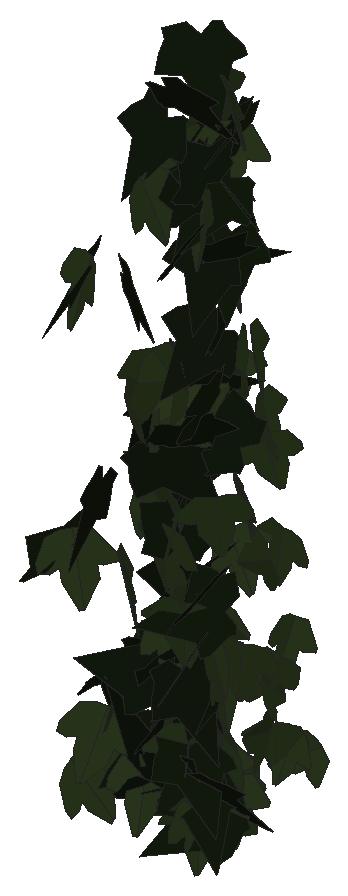
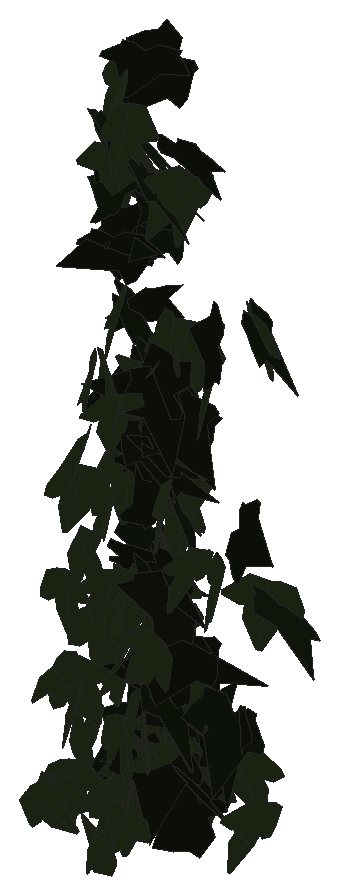
# SketchUp Ruby script. Lengths in inches.
U = 1.inch
M = Sketchup.active_model
def pt(a) = Geom::Point3d.new(a.map { |v| v * U })
def face(e, loops, mat)
  f = e.add_face(loops[0].map { |a| pt(a) })
  loops[1..].each { |l| e.add_face(l.map { |a| pt(a) }).erase! }
  f.material = f.back_material = mat if mat
  f
end
# faces: each face lists its corners as indices into pts; further lists are holes
def faces(e, pts, list, mat = nil) = list.each { |f| face(e, (f[0].is_a?(Array) ? f : [f]).map { |l| l.map { |i| pts[i] } }, mat) }
# xy, xz, yz: faces in a plane at the given z, y or x. An outline is a flat list of corners, or four numbers for a rectangle; further outlines are holes
def ring(l) = l.size == 4 ? [[l[0], l[1]], [l[2], l[1]], [l[2], l[3]], [l[0], l[3]]] : l.each_slice(2).to_a
def flat(e, list, mat, &to3) = list.each { |f| face(e, (f[0].is_a?(Array) ? f : [f]).map { |l| ring(l).map { |u, v| to3.(u, v) } }, mat) }
def xy(e, z, list, mat = nil) = flat(e, list, mat) { |x, y| [x, y, z] }
def xz(e, y, list, mat = nil) = flat(e, list, mat) { |x, z| [x, y, z] }
def yz(e, x, list, mat = nil) = flat(e, list, mat) { |y, z| [x, y, z] }
def lines(e, pts, list) = list.each { |a, b| e.add_line(pt(pts[a]), pt(pts[b])) }
# prism: a flat outline (further loops are holes) pulled along v
def prism(e, loops, v, mat = nil)
  f = face(e, loops, mat); d = Geom::Vector3d.new(v.map { |x| x * U })
  f.pushpull(f.normal.samedirection?(d) ? d.length : -d.length)
end
def box(e, o, s, mat = nil) = prism(e, [[o, [o[0] + s[0], o[1], o[2]], [o[0] + s[0], o[1] + s[1], o[2]], [o[0], o[1] + s[1], o[2]]]], [0, 0, s[2]], mat)
def at(x, y, z, deg = 0) = Geom::Transformation.translation(pt([x, y, z])) * Geom::Transformation.rotation(ORIGIN, Z_AXIS, deg.degrees)
def axes(o, x, y, z) = Geom::Transformation.new([*x, 0, *y, 0, *z, 0, *pt(o).to_a, 1])
def part(name) = M.definitions.add(name)
# library, detail: a bought-in or finely detailed component or shape, given as its bounding box
def library(name, o, s) = part(name).tap { |d| box(d.entities, o, s) }
def detail(e, o, s) = box(e.add_group.entities, o, s)
def put(e, d, t, mat = nil) = e.add_instance(d, t).tap { |i| i.material = mat if mat }
def group(e, t, mat = nil) = e.add_group.tap { |g| g.transformation = t; g.material = mat if mat }.entities
root = M.entities
M.materials.add("efeu1").color = [18, 25, 13]
M.materials.add("efeu2").color = [43, 57, 29]
c1 = part("ivyleaf_9")
p = [[1.54,2.16,1.25],[1.36,2.04,1.19],[-0.21,0.99,0.68],[-0.71,1.11,0.82],[-0.85,0.86,0.67],[-0.8,0.17,0.21],
  [-0.9,-0.01,0.1],[-0.67,-0.16,-0.02],[-0.08,-0.08,-0.05],[-0.03,-0.6,-0.4],[0.65,-0.88,-0.66],[0.83,-0.6,-0.49],
  [1.29,-0.42,-0.43],[1.8125,-0.07,-0.26],[1.21,0.44,0.15]]
faces(c1.entities,p,[[0,1,2,3,4,5,6,7,8,9,10,11,12,13,14]],"efeu1")
c2 = part("ivyleaf_10")
p = [[0,0.5,-0.03],[-0.0625,2.02,-0.43],[-0.19,2.01,-0.46],[-0.54,1.05,-0.29],[-0.52,0.625,-0.18],[-0.83,0.76,-0.28],
  [-1.16,0.64,-0.33],[-1.15,0.33,-0.24],[-0.77,-0.39,0.02],[-0.3,-0.51,0.16],[0.04,-0.48,0.23],[-0.02,2.01,-0.4375],
  [-0.06,2.01,-0.43],[0.04,-0.49,0.23],[0.67,-0.49,0.14],[1.38,0.36,-0.2],[1.375,0.51,-0.24],[0.81,0.65,-0.19],
  [0.62,0.59,-0.15],[0.6,1.09,-0.28],[0.5,1.23,-0.31]]
faces(c2.entities,p,[[0,1,2,3,4,5,6,7,8,9,10],[11,12,0,13,14,15,16,17,18,19,20]],"efeu2")
put(root,c1,axes([599.48,135.08,196.09],[-0.17515,0.56186,0.50454],[-0.19533,0.4666,-0.58741],[-0.72945,-0.25986,0.03615]))
put(root,c2,axes([598.03,135.5,191.97],[-0.83142,0.16967,0.09937],[-0.11258,-0.05682,-0.845],[-0.1612,-0.83541,0.07765]))
put(root,c2,axes([597.29,135.13,195.71],[-0.33542,0.39582,0.64097],[-0.41193,0.49108,-0.51882],[-0.63074,-0.53122,-0.00202]))
put(root,c1,axes([598.03,135.34,194.51],[-0.09921,-0.26302,-0.75239],[0.1878,0.72913,-0.27966],[0.77459,-0.21047,-0.02857]))
put(root,c1,axes([598.74,135.27,195.4],[0.4239,0.64776,-0.12364],[-0.07765,-0.09693,-0.77404],[-0.65486,0.43079,0.01175]))
put(root,c1,axes([598.58,135.89,185.9375],[0.02815,-0.77163,-0.17513],[0.1769,0.17695,-0.75118],[0.77123,-0.01242,0.1787]))
put(root,c2,axes([597.77,135.55,196.91],[-0.60445,-0.48908,-0.20865],[0.17064,0.12078,-0.77743],[0.50361,-0.62794,0.01298]))
put(root,c1,axes([598.28,135.375,204.74],[0.79843,0.15118,0.0487],[0.04798,0.00835,-0.81262],[-0.15141,0.79987,-0.00073]))
put(root,c1,axes([597.47,135.74,187.67],[-0.46495,0.1516,0.60854],[-0.58334,0.17358,-0.48894],[-0.23025,-0.7459,0.0099]))
put(root,c1,axes([599.15,135.2,190.59],[-0.05658,0.74396,0.27596],[-0.0347,0.27407,-0.746],[-0.79273,-0.06509,0.01296]))
put(root,c2,axes([597.77,135.15,196.43],[-0.10669,-0.23752,-0.78971],[0.33307,0.71605,-0.26036],[0.75441,-0.34972,0.00326]))
put(root,c1,axes([595.51,136.1,192.29],[-0.21723,0.20492,-0.73112],[0.53933,-0.49364,-0.2986],[-0.53447,-0.58142,-0.00416]))
put(root,c2,axes([597.76,136.12,190.25],[0.214,-0.2507,-0.71753],[0.44642,-0.56185,0.32945],[-0.61515,-0.49495,-0.01054]))
put(root,c1,axes([598.64,135.09,188.23],[0.12071,0.46617,0.65874],[0.01962,0.66418,-0.47361],[-0.80676,0.0859,0.08704]))
put(root,c2,axes([595.14,135.88,198.32],[0.69254,-0.41807,0.0234],[0.02287,-0.00739,-0.80893],[0.4181,0.6929,0.0055]))
put(root,c1,axes([598.91,136.32,197.7],[-0.39809,-0.60806,0.27911],[-0.14546,-0.23836,-0.72674],[0.65306,-0.42375,0.00827]))
put(root,c2,axes([598.62,135.35,196.51],[0.0499,-0.09413,-0.86374],[-0.53865,0.67548,-0.10473],[0.68173,0.54061,-0.01953]))
put(root,c1,axes([595.23,135.91,198.4],[-0.585,0.44066,-0.32599],[0.25378,-0.20485,-0.73233],[-0.48584,-0.6376,0.00999]))
put(root,c2,axes([598.9,135.93,184.54],[-0.25955,-0.79481,0.09066],[-0.00821,-0.09266,-0.83586],[0.79992,-0.25884,0.02083]))
put(root,c1,axes([599.375,136,190.09],[-0.69551,0.10376,0.4092],[-0.41383,-0.01181,-0.70039],[-0.08338,-0.80687,0.06287]))
put(root,c1,axes([598.72,136.06,184.94],[-0.06841,-0.75084,-0.2086],[0.16447,0.19078,-0.74061],[0.76172,-0.10862,0.14118]))
put(root,c2,axes([598.46,135.8,189.77],[-0.77585,-0.31539,0.09171],[-0.075,-0.05893,-0.83709],[0.31977,-0.77902,0.02619]))
put(root,c2,axes([598.9375,135.75,184.42],[0.31576,0.78872,-0.0383],[-0.1311,0.01168,-0.84019],[-0.77869,0.31786,0.12592]))
put(root,c2,axes([598.68,136.05,201.31],[0.63049,-0.31526,0.33383],[0.2973,-0.15187,-0.70491],[0.34992,0.69706,-0.00259]))
put(root,c2,axes([597.98,135.73,192.43],[0.49156,-0.52468,-0.39049],[-0.26546,0.28639,-0.71897],[0.59775,0.55866,0.00183]))
put(root,c2,axes([598.41,135.92,186.31],[-0.44957,-0.657,0.04508],[0.04346,-0.08407,-0.79173],[0.65711,-0.44393,0.08321]))
put(root,c2,axes([594.93,135.72,190.5],[0.7318,0.39439,0.16682],[0.07748,0.20292,-0.81959],[-0.42115,0.72263,0.1391]))
put(root,c1,axes([599.31,136.27,184.27],[-0.69308,-0.25006,0.34141],[-0.3081,-0.15097,-0.73603],[0.29011,-0.75772,0.03397]))
put(root,c2,axes([596.51,135.82,190.39],[-0.53032,0.65007,-0.14118],[0.06273,-0.13088,-0.83827],[-0.66226,-0.53296,0.03365]))
put(root,c1,axes([598.33,135.89,187.99],[0.16995,-0.72031,-0.40589],[-0.09788,0.39394,-0.74007],[0.82098,0.19607,-0.00421]))
put(root,c2,axes([598.01,135.7,192.46],[-0.30314,0.13366,-0.74242],[-0.67019,0.31957,0.33117],[0.34628,0.7355,-0.00897]))
put(root,c1,axes([597.74,135.98,184.44],[0.55605,-0.4331,0.90783],[-0.70662,0.57003,0.70476],[-0.71583,-0.89912,0.00951]))
put(root,c2,axes([597.35,135.65,201.41],[0.02179,0.75819,0.25552],[-0.04629,0.25638,-0.7568],[-0.79875,0.00582,0.05083]))
put(root,c2,axes([598.02,136.11,185.84],[0.6614,-0.50269,0.10098],[0.08148,-0.05968,-0.83075],[0.50622,0.6664,0.00177]))
put(root,c2,axes([597.89,135.92,195.04],[0.12927,0.79092,-0.04758],[-0.01141,-0.04634,-0.8014],[-0.79227,0.12971,0.00378]))
put(root,c2,axes([596.87,136.05,184.62],[0.79945,0.05348,0.06015],[0.06007,0.00311,-0.80124],[-0.05357,0.80171,-0.0009]))
put(root,c2,axes([598.08,135.74,195.3125],[0.44704,0.04825,-0.66928],[0.64371,0.19622,0.44411],[0.18945,-0.78056,0.07027]))
put(root,c1,axes([598.49,135.35,200.05],[0.17816,0.49731,0.59196],[0.07371,0.59378,-0.52102],[-0.76961,0.17199,0.08713]))
put(root,c2,axes([595.47,136.13,185.53],[0.77809,0.23006,-0.17094],[-0.16674,-0.03892,-0.81133],[-0.23312,0.7957,0.00974]))
put(root,c1,axes([598.34,135.72,191.85],[-0.41721,-0.32068,0.67833],[0.53805,0.41307,0.52621],[-0.52294,0.68085,0.00024]))
put(root,c2,axes([599.2,136.0625,192.94],[-0.57017,-0.53486,-0.04718],[0.03496,0.0317,-0.78178],[0.5358,-0.57124,0.0008]))
put(root,c1,axes([597.87,135.91,186.68],[-0.27729,0.78448,-0.14614],[0.06048,-0.1336,-0.83195],[-0.79568,-0.28354,-0.01231]))
put(root,c1,axes([598.78,136.51,199.88],[-0.2675,-0.71367,0.01173],[-0.0042,-0.01096,-0.76215],[0.71375,-0.26753,-0.00009]))
put(root,c2,axes([597.36,136.02,187.1],[-0.74119,0.1043,-0.17165],[0.17063,-0.01923,-0.74848],[-0.10596,-0.76056,-0.00461]))
put(root,c1,axes([599.14,135.71,202.32],[-0.13653,0.53416,0.54564],[-0.41867,0.41118,-0.50728],[-0.63856,-0.38379,0.21593]))
put(root,c1,axes([594.48,135.73,190.2],[-0.24482,0.73594,0.3292],[-0.32043,0.22688,-0.7455],[-0.7398,-0.34181,0.21396]))
put(root,c1,axes([598.68,135.99,201.83],[-0.51041,0.43494,0.41114],[-0.35354,0.21689,-0.66835],[-0.48292,-0.61848,0.05475]))
put(root,c1,axes([597.25,136.46,203.02],[-0.71954,-0.19735,-0.20147],[0.20001,0.03213,-0.74581],[0.19882,-0.74652,0.02116]))
put(root,c1,axes([598.75,135.8,185.07],[0.82989,0.15234,0.10307],[0.08699,0.09458,-0.84026],[-0.16206,0.8309,0.07675]))
put(root,c2,axes([599.08,136.03,189.03],[-0.2248,0.70811,0.06754],[-0.01675,0.06554,-0.74293],[-0.71113,-0.22539,-0.00385]))
put(root,c1,axes([597.89,135.75,192.38],[-0.28954,0.59237,0.494],[-0.19526,0.45418,-0.65907],[-0.7462,-0.3487,-0.01922]))
put(root,c2,axes([597.64,136.22,189.02],[0.36369,0.69944,-0.01687],[-0.00786,-0.01492,-0.78834],[-0.6996,0.36377,0.00009]))
put(root,c2,axes([595.05,135.89,184.05],[0.09385,0.7266,0.41294],[0.04741,0.41024,-0.73262],[-0.8344,0.10504,0.00482]))
put(root,c1,axes([598.66,136.4,187.22],[-0.72112,0.37351,-0.01669],[-0.04987,-0.13203,-0.79993],[-0.37054,-0.70913,0.14014]))
put(root,c2,axes([597.77,136.02,190.68],[-0.57427,0.4899,0.28609],[-0.22552,0.17641,-0.75476],[-0.52056,-0.61686,0.01137]))
put(root,c2,axes([597.76,136.26,186.46],[-0.10204,0.73817,-0.0861],[0.00139,-0.08672,-0.74512],[-0.74318,-0.10152,0.01042]))
put(root,c1,axes([599,136.72,201.83],[-0.67768,-0.409,-0.01842],[0.01637,0.00852,-0.79154],[0.40909,-0.67788,0.00117]))
put(root,c1,axes([597.48,136.37,195.17],[-0.03756,0.59258,-0.4817],[-0.12238,-0.48072,-0.58183],[-0.7538,0.04852,0.11847]))
put(root,c1,axes([598.99,136.58,197.98],[-0.59621,0.31029,-0.35451],[0.27458,-0.23579,-0.66816],[-0.38284,-0.65234,0.07288]))
put(root,c1,axes([598.08,136.25,190.4],[-0.16878,0.01522,-0.77787],[-0.76448,-0.15106,0.16292],[-0.14448,0.7815,0.04664]))
put(root,c1,axes([598.17,136.32,193.31],[-0.43099,0.24942,0.60677],[-0.52164,0.30999,-0.49794],[-0.39785,-0.67664,-0.00445]))
put(root,c1,axes([595.75,136.15,186.64],[0.45284,0.09373,-0.6358],[-0.64167,0.02251,-0.4537],[-0.03588,0.78026,0.08946]))
put(root,c1,axes([599.38,136.63,194.51],[-0.23304,0.09191,0.72797],[-0.73365,-0.01646,-0.23278],[-0.01222,-0.76418,0.09257]))
put(root,c1,axes([597.4,136.03,187.26],[0.26049,0.06632,0.71485],[0.65229,0.29578,-0.26514],[-0.29988,0.70099,0.04424]))
put(root,c1,axes([598.5,136.6,185.51],[-0.72874,0.30952,0.03809],[-0.0838,-0.1011,-0.78171],[-0.30039,-0.72269,0.12567]))
put(root,c1,axes([597.17,136.04,188.47],[0.66728,0.50259,0.04955],[0.04373,0.02431,-0.83535],[-0.50313,0.66867,-0.00688]))
put(root,c1,axes([595.76,136.78,197.875],[0.20868,-0.06172,-0.74778],[0.74688,-0.05708,0.21315],[-0.07169,-0.77425,0.04389]))
put(root,c1,axes([596.57,136.3,183.66],[0.48787,0.58664,-0.32179],[0.21106,0.24299,0.76297],[0.63494,-0.53153,-0.00636]))
put(root,c1,axes([598.18,136.71,205.57],[-0.28676,-0.5517,-0.47132],[0.3021,0.37,-0.61691],[0.65973,-0.40923,0.07762]))
put(root,c2,axes([599.05,136.66,184.18],[0.47922,-0.00739,-0.60101],[-0.60031,0.03252,-0.47905],[0.03003,0.76799,0.0145]))
put(root,c2,axes([598.49,136.8,189.56],[-0.11099,0.04369,-0.73699],[0.65061,-0.34649,-0.11853],[-0.34897,-0.65987,0.01344]))
put(root,c1,axes([597.85,136.42,195.88],[-0.00056,0.76781,-0.18396],[0.00633,-0.18395,-0.76779],[-0.78952,-0.00202,-0.00602]))
put(root,c2,axes([595.67,136.48,185.62],[0.25176,-0.65765,0.35181],[-0.1295,0.32712,0.70418],[-0.73451,-0.28309,-0.00357]))
put(root,c2,axes([598.28,137.11,184],[-0.2401,0.20508,0.71295],[0.53247,-0.47415,0.31571],[0.51657,0.58406,0.00595]))
put(root,c2,axes([598.26,136.77,184.53],[-0.5946,-0.16977,0.33654],[-0.30668,-0.14756,-0.61628],[0.21915,-0.66711,0.05067]))
put(root,c1,axes([597.75,136.5,187.15],[-0.37506,0.71976,-0.00582],[-0.00081,-0.00699,-0.81161],[-0.71979,-0.37504,0.00395]))
put(root,c1,axes([597.43,136.19,189.52],[-0.06163,0.78621,-0.26039],[-0.02428,0.25928,0.78861],[0.82785,0.06614,0.00375]))
put(root,c1,axes([597.59,136.42,195.69],[0.3779,0.04918,0.66035],[0.65023,0.11624,-0.38076],[-0.12524,0.7519,0.01567]))
put(root,c2,axes([597.29,136.74,185.47],[0.42994,0.68079,-0.01207],[-0.04069,0.01144,-0.80417],[-0.67968,0.42996,0.0405]))
put(root,c1,axes([598.25,136.81,194.77],[-0.36857,0.59985,-0.325],[0.17966,-0.27102,-0.70396],[-0.65816,-0.4099,-0.01017]))
put(root,c2,axes([599,136.73,204.46],[-0.57255,0.54729,-0.1407],[0.1116,-0.08684,-0.79192],[-0.55395,-0.58315,-0.01411]))
put(root,c1,axes([598.8,136.25,199.6875],[0.44997,0.29569,0.54471],[0.40899,0.36412,-0.5355],[-0.4657,0.60548,0.05602]))
put(root,c1,axes([596.6875,136.92,184.98],[-0.76098,0.23429,0.0636],[-0.06777,-0.00408,-0.79587],[-0.23312,-0.76362,0.02377]))
put(root,c1,axes([598.83,137.07,200.05],[-0.41992,-0.53417,-0.34372],[0.28547,0.20938,-0.67415],[0.56744,-0.50064,0.08479]))
put(root,c2,axes([599.45,136.8,188.59],[-0.72286,-0.31484,0.13087],[-0.12968,-0.02985,-0.78808],[0.31533,-0.734,-0.02408]))
put(root,c2,axes([598.83,136.83,185.57],[-0.71162,0.2824,0.22154],[-0.2777,-0.12153,-0.73712],[-0.2274,-0.73534,0.2069]))
put(root,c2,axes([598.74,136.83,183.77],[-0.69527,-0.32853,0.09744],[-0.09468,-0.02766,-0.76883],[0.32934,-0.70152,-0.01532]))
put(root,c1,axes([599.03,136.87,203.24],[-0.5316,0.55983,-0.11159],[0.02452,-0.12995,-0.76875],[-0.57032,-0.52742,0.07097]))
put(root,c1,axes([595.61,136.37,186.96],[0.17098,0.77501,0.18738],[-0.06267,0.20411,-0.78701],[-0.79487,0.15061,0.10236]))
put(root,c2,axes([599,136.47,188.35],[0.23411,-0.2473,0.67716],[-0.41935,0.53241,0.33941],[-0.58639,-0.47948,0.02762]))
put(root,c2,axes([598.68,136.95,187.62],[-0.09386,0.71736,-0.13127],[0.02188,-0.12953,-0.72346],[-0.72894,-0.09626,-0.00481]))
put(root,c1,axes([598.42,137.125,193.93],[-0.54657,0.07563,0.53038],[-0.5292,0.04185,-0.55132],[-0.08348,-0.76045,0.0224]))
put(root,c1,axes([598.375,137.32,201.66],[0.28736,-0.59697,0.37739],[0.31687,-0.25515,-0.64488],[0.63119,0.39987,0.15193]))
put(root,c1,axes([597.51,136.78,185.42],[0.47694,0.59197,-0.27746],[-0.1797,-0.21151,-0.76016],[-0.62858,0.50962,0.0068]))
put(root,c1,axes([599.21,136.89,203.1],[-0.52163,0.58354,0.14992],[-0.12065,0.09311,-0.78222],[-0.59028,-0.5347,0.0274]))
put(root,c2,axes([597.03,136.62,201.99],[0.18245,0.50471,0.55421],[-0.00471,0.57115,-0.51859],[-0.74957,0.11926,0.13815]))
put(root,c2,axes([597.58,136.76,184.92],[0.26218,0.23896,0.72676],[0.47978,0.54704,-0.35295],[-0.5959,0.54559,0.03558]))
put(root,c1,axes([597.83,137.22,202.49],[-0.58959,0.46986,-0.10387],[0.07037,-0.07832,-0.75372],[-0.47603,-0.59353,0.01723]))
put(root,c2,axes([598.76,137.34,184.25],[0.2534,0.66378,-0.21334],[-0.0742,-0.20003,-0.7105],[-0.69326,0.26404,-0.00193]))
put(root,c2,axes([598.03,136.97,186.22],[-0.26313,0.25906,0.61267],[-0.53848,0.30386,-0.35975],[-0.39053,-0.59352,0.08324]))
put(root,c2,axes([598.61,137.32,202.68],[0.69781,0.33472,-0.03971],[-0.06666,0.04755,-0.77062],[-0.33041,0.69732,0.07161]))
put(root,c2,axes([598.26,137.3,203.84],[-0.17311,-0.68298,-0.32534],[0.07142,0.3175,-0.70453],[0.75313,-0.1871,-0.00797]))
put(root,c2,axes([596.13,137.17,191.64],[0.02543,0.66229,0.34031],[0.02681,0.33947,-0.66267],[-0.74413,0.03487,-0.01224]))
put(root,c2,axes([598.41,137.32,185.86],[-0.51659,0.21566,0.42487],[-0.40747,0.12486,-0.55881],[-0.24697,-0.6571,0.03326]))
put(root,c2,axes([599.02,137.34,196.22],[-0.07579,0.14577,0.74173],[-0.70443,0.25678,-0.12244],[-0.27419,-0.69998,0.10955]))
put(root,c2,axes([599.08,138.17,185.58],[-0.01251,-0.23978,-0.66077],[0.00198,-0.66088,0.23978],[-0.70293,0.0024,0.01243]))
put(root,c2,axes([599.6,137.51,190.96],[-0.31382,0.04141,0.63783],[-0.63424,0.06795,-0.31647],[-0.07928,-0.7076,0.00693]))
put(root,c2,axes([598.71,137.65,192.52],[-0.5318,0.49186,-0.02565],[0.02107,-0.015,-0.72439],[-0.49208,-0.53221,-0.00329]))
put(root,c2,axes([596.9,137.88,189.05],[-0.5833,0.11038,-0.40021],[0.38001,-0.13593,-0.59136],[-0.16716,-0.69421,0.05216]))
put(root,c2,axes([596.79,137.58,193.54],[-0.44486,0.42017,0.38541],[-0.26324,0.28226,-0.61157],[-0.50575,-0.5165,-0.02069]))
put(root,c2,axes([598.08,137.85,195.81],[0.32317,0.63237,0.11758],[0.00806,0.12759,-0.70839],[-0.64316,0.31935,0.0502]))
put(root,c2,axes([598.13,137.8,198.75],[-0.34993,0.64337,0.15248],[-0.08464,0.12751,-0.73226],[-0.65575,-0.35978,0.01314]))
put(root,c2,axes([599.35,138.21,187.61],[-0.48355,-0.33267,0.38508],[-0.31097,-0.22731,-0.58686],[0.40281,-0.57483,0.00921]))
put(root,c2,axes([598.82,138.08,196.67],[-0.33485,0.64099,-0.09276],[0.00235,-0.10322,-0.72176],[-0.64766,-0.33177,0.04534]))
put(root,c2,axes([598.21,137.98,190.74],[0.23772,0.63936,0.18485],[0.08084,0.16709,-0.68191],[-0.66061,0.25051,-0.01693]))
put(root,c2,axes([597.44,138.4,184.24],[0.59552,0.1688,0.28357],[0.26977,0.08796,-0.61889],[-0.19007,0.65369,0.01006]))
put(root,c2,axes([598.94,138.42,193.6],[-0.48738,-0.48443,-0.14762],[0.13841,0.06966,-0.68556],[0.48714,-0.50445,0.04709]))
put(root,c2,axes([598.89,138.37,194.65],[-0.19732,0.68446,0.04343],[-0.00931,0.04251,-0.71233],[-0.68577,-0.19752,-0.00282]))
put(root,c2,axes([599.25,138.08,187.07],[-0.20693,0.39976,0.54185],[-0.30563,0.44934,-0.44822],[-0.59999,-0.36676,0.04145]))
put(root,c2,axes([597.85,138.97,183.78],[-0.04306,0.44145,-0.49501],[-0.06989,-0.49631,-0.43653],[-0.65957,0.02377,0.07857]))
put(root,c2,axes([597.66,138.88,183.26],[0.22007,-0.13751,-0.61151],[0.50804,-0.34043,0.25939],[-0.36707,-0.55361,-0.00761]))
put(root,c2,axes([599.21,139.04,188.18],[0.13413,0.55805,-0.35439],[-0.10751,-0.33838,-0.57353],[-0.65226,0.17053,0.02166]))
put(root,c2,axes([598.91,138.87,185.25],[-0.54806,-0.33572,0.07291],[-0.06951,-0.02607,-0.64256],[0.33644,-0.55227,-0.01399]))
put(root,c2,axes([599.04,138.91,190.77],[-0.66611,0.06782,0.13447],[-0.1451,-0.12568,-0.65539],[-0.04034,-0.66783,0.137]))
put(root,c2,axes([599.05,139.14,184.96],[0.63107,-0.04681,-0.10964],[-0.10789,0.02705,-0.63253],[0.05072,0.63995,0.01871]))
put(root,c2,axes([599.39,139.52,184.6],[0.36844,0.03784,-0.52875],[-0.53008,0.0313,-0.36714],[0.00412,0.6437,0.04893]))
